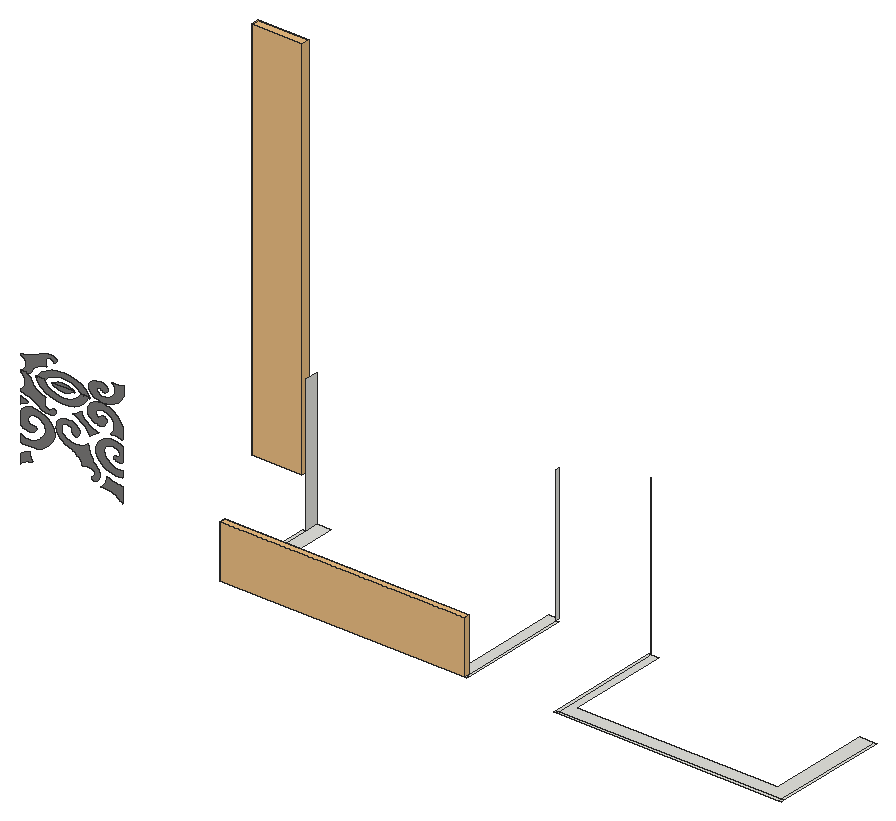
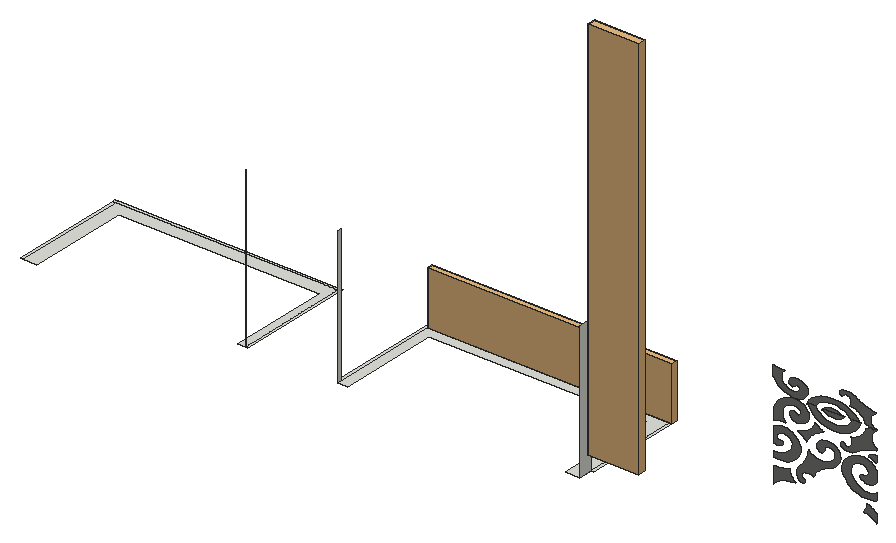
# SketchUp Ruby script. Lengths in inches.
U = 1.inch
M = Sketchup.active_model
def pt(a) = Geom::Point3d.new(a.map { |v| v * U })
def face(e, loops, mat)
  f = e.add_face(loops[0].map { |a| pt(a) })
  loops[1..].each { |l| e.add_face(l.map { |a| pt(a) }).erase! }
  f.material = f.back_material = mat if mat
  f
end
# faces: each face lists its corners as indices into pts; further lists are holes
def faces(e, pts, list, mat = nil) = list.each { |f| face(e, (f[0].is_a?(Array) ? f : [f]).map { |l| l.map { |i| pts[i] } }, mat) }
# xy, xz, yz: faces in a plane at the given z, y or x. An outline is a flat list of corners, or four numbers for a rectangle; further outlines are holes
def ring(l) = l.size == 4 ? [[l[0], l[1]], [l[2], l[1]], [l[2], l[3]], [l[0], l[3]]] : l.each_slice(2).to_a
def flat(e, list, mat, &to3) = list.each { |f| face(e, (f[0].is_a?(Array) ? f : [f]).map { |l| ring(l).map { |u, v| to3.(u, v) } }, mat) }
def xy(e, z, list, mat = nil) = flat(e, list, mat) { |x, y| [x, y, z] }
def xz(e, y, list, mat = nil) = flat(e, list, mat) { |x, z| [x, y, z] }
def yz(e, x, list, mat = nil) = flat(e, list, mat) { |y, z| [x, y, z] }
def lines(e, pts, list) = list.each { |a, b| e.add_line(pt(pts[a]), pt(pts[b])) }
# prism: a flat outline (further loops are holes) pulled along v
def prism(e, loops, v, mat = nil)
  f = face(e, loops, mat); d = Geom::Vector3d.new(v.map { |x| x * U })
  f.pushpull(f.normal.samedirection?(d) ? d.length : -d.length)
end
def box(e, o, s, mat = nil) = prism(e, [[o, [o[0] + s[0], o[1], o[2]], [o[0] + s[0], o[1] + s[1], o[2]], [o[0], o[1] + s[1], o[2]]]], [0, 0, s[2]], mat)
def at(x, y, z, deg = 0) = Geom::Transformation.translation(pt([x, y, z])) * Geom::Transformation.rotation(ORIGIN, Z_AXIS, deg.degrees)
def axes(o, x, y, z) = Geom::Transformation.new([*x, 0, *y, 0, *z, 0, *pt(o).to_a, 1])
def part(name) = M.definitions.add(name)
# library, detail: a bought-in or finely detailed component or shape, given as its bounding box
def library(name, o, s) = part(name).tap { |d| box(d.entities, o, s) }
def detail(e, o, s) = box(e.add_group.entities, o, s)
def put(e, d, t, mat = nil) = e.add_instance(d, t).tap { |i| i.material = mat if mat }
def group(e, t, mat = nil) = e.add_group.tap { |g| g.transformation = t; g.material = mat if mat }.entities
root = M.entities
M.materials.add("[0043_SaddleBrown]4").color = [124, 123, 122]
M.materials.add("[Granite Light Gray]").color = [149, 148, 144]
c1 = library("Scandinavian Door w/ Glass Wall\#2",[-41.94,78.85,0],[6.47,62.99,82.68])
c2 = library("Glass Railing",[0,0,0],[139.5,4.76,42])
xy(root,413.5,[[550.01,557.9375,742.44,559.875],[742.44,557.9375,744.38,559.875],[812.96,557.9375,814.89,559.875],[814.89,557.9375,990.19,559.875],[990.19,557.9375,992.12,559.875],
  [549.82,559.875,551.76,640.11],[551.76,559.875,742.44,559.875,742.44,651.03,734.59,651.03,734.59,570.83,563.08,570.83,563.08,651.03,551.76,651.03],[742.44,559.875,744.38,647.91],[812.96,559.875,814.89,651.03],[814.89,559.875,990.19,559.875,990.19,651.03,978.86,651.03,978.86,570.83,820.97,570.83,820.97,651.03,814.89,651.03],
  [990.19,559.875,992.12,651.03]])
xz(root,589.17,[[448.37,418.4,448.37,430.94,447.33,430.96,446.29,431.01,445.26,431.09,444.23,431.2,443.21,431.34,442.2,431.51,441.19,431.7,440.2,431.93,439.22,432.18,438.26,432.46,437.3125,432.77,436.38,433.11,436.28,432.33,436.12,431.56,435.91,430.79,435.64,430.03,435.32,429.29,434.95,428.55,434.53,427.83,434.05,427.13,433.53,426.44,432.96,425.78,432.34,425.14,431.68,424.52,433.34,424.625,435,424.61,436.65,424.48,438.27,424.22,439.85,423.85,441.36,423.36,442.8,422.76,444.15,422.0625,445.39,421.27,446.52,420.39,447.51,419.43],[367.98,418.5,368.5,419.14,369.09,419.74,369.74,420.3125,370.46,420.84,371.24,421.32,372.07,421.76,372.94,422.14,373.86,422.48,374.81,422.75,375.78,422.98,376.78,423.14,377.8,423.24,377.38,423.73,377,424.24,376.65,424.76,376.35,425.29,376.08,425.83,375.85,426.38,375.66,426.94,375.51,427.51,375.4,428.08,375.33,428.65,375.3,429.23,375.32,429.8,374.62,429.54,373.94,429.27,373.26,428.97,372.61,428.66,371.97,428.33,371.34,427.99,370.73,427.63,370.14,427.26,369.57,426.87,369.02,426.47,368.49,426.05,367.98,425.62],[426.05,427.2,426.61,427.23,427.15,427.32,427.68,427.46,428.16,427.66,428.61,427.9,429,428.18,429.33,428.51,429.6,428.86,429.79,429.24,429.91,429.63,429.94,430.04,430.16,430.71,430.3,431.38,430.38,432.07,430.39,432.76,430.32,433.44,430.19,434.125,429.99,434.8,429.73,435.46,429.39,436.1,428.99,436.72,428.54,437.33,428.02,437.9,427.08,438.91,426.21,439.95,425.41,441.02,424.67,442.11,424,443.22,423.41,444.36,422.88,445.51,422.43,446.68,422.05,447.86,421.75,449.05,421.52,450.26,421.37,451.46,420.4,450.57,419.28,449.77,418.03,449.08,416.66,448.52,415.2,448.09,413.68,447.8,412.12,447.66,410.54,447.66,408.98,447.8125,407.46,448.11,406.01,448.54,404.64,449.11,403.67,449.65,402.8,450.27,402.05,450.97,401.43,451.74,400.95,452.55,400.625,453.4,400.45,454.28,400.43,455.16,400.57,456.04,400.87,456.9,401.32,457.72,401.91,458.5,402.45,458.79,403.06,459.03,403.7,459.19,404.37,459.29,405.05,459.31,405.73,459.26,406.39,459.13,407.02,458.94,407.6,458.68,408.12,458.36,408.57,457.99,408.9375,457.57,408.82,457.28,408.73,456.98,408.68,456.67,408.66,456.37,408.67,456.06,408.72,455.75,408.8,455.45,408.91,455.16,409.06,454.87,409.24,454.59,409.45,454.32,409.68,454.0625,409.91,453.87,410.1875,453.7,410.49,453.5625,410.82,453.47,411.17,453.41,411.53,453.38,411.89,453.41,412.23,453.47,412.57,453.5625,412.87,453.7,413.14,453.87,413.375,454.0625,414.05,454.87,414.52,455.75,414.78,456.67,414.8125,457.61,414.625,458.54,414.22,459.4375,413.6,460.27,412.8,461.01,411.84,461.64,410.74,462.15,409.53,462.51,408.26,462.72,406.84,462.91,405.4,462.94,403.96,462.8125,402.58,462.53,401.26,462.1,400.05,461.53,398.98,460.83,398.07,460.03,397.33,459.13,396.79,458.17,396.47,457.15,396.36,456.12,396.24,454.92,396.31,453.72,396.54,452.53,396.94,451.37,397.51,450.24,398.24,449.16,399.12,448.14,400.14,447.19,401.29,446.32,402.56,445.55,403.93,444.87,405.4,444.3,406.79,443.78,408.12,443.1875,409.39,442.53,410.6,441.81,411.73,441.03,412.78,440.19,413.74,439.31,414.62,438.37,415.4,437.39,416.09,436.38,416.67,435.33,417.15,434.26,417.83,434.625,418.57,434.93,419.36,435.15,420.18,435.3,421.03,435.36,421.88,435.34,422.72,435.24,423.53,435.05,424.3,434.79,425.01,434.46,425.65,434.06,426.22,433.6,426.42,433.23,426.57,432.84,426.65,432.45,426.68,432.05,426.64,431.65,426.53,431.26,426.37,430.875,426.15,430.51,425.875,430.16,425.54,429.84,425.17,429.55,424.75,429.29,424.52,429.13,424.33,428.95,424.2,428.75,424.13,428.53,424.12,428.3,424.17,428.08,424.28,427.87,424.44,427.67,424.65,427.51,424.91,427.375,425.19,427.28,425.5,427.23],[374.59,433.3,376.85,433.36,379.09,433.62,381.26,434.07,383.35,434.7,385.3125,435.5,387.13,436.47,388.77,437.59,390.22,438.85,391.45,440.22,393.12,442.26,394.27,444.47,394.89,446.8,394.93,449.17,394.41,451.51,393.34,453.75,391.75,455.82,389.6875,457.67,387.21,459.23,384.41,460.46,381.35,461.32,378.13,461.79,376.97,461.63,375.83,461.4,374.74,461.08,373.6875,460.69,372.69,460.24,371.76,459.71,370.91,459.125,370.13,458.48,369.45,457.79,368.86,457.06,368.36,456.28,367.98,455.48,367.98,447.4,368.51,446.49,369.28,445.68,370.27,445,371.43,444.48,372.71,444.15,374.05,444,375.42,444.0625,376.73,444.32,377.95,444.76,379.01,445.37,379.88,446.13,380.52,447,380.62,447.21,380.67,447.42,380.67,447.64,380.63,447.86,380.55,448.07,380.42,448.27,380.26,448.46,380.06,448.62,379.82,448.76,379.57,448.88,379.29,448.97,378.99,449.02,378.26,448.93,377.53,448.94,376.81,449.05,376.125,449.25,375.5,449.54,374.97,449.9,374.53,450.33,374.22,450.81,374.03,451.32,373.97,451.85,374.06,452.38,374.27,452.89,374.45,453.55,374.78,454.18,375.24,454.77,375.82,455.29,376.51,455.75,377.28,456.12,378.13,456.4,379.03,456.57,379.96,456.65,380.89,456.62,381.81,456.48,382.68,456.24,384.03,455.45,385.22,454.53,386.22,453.51,387,452.39,387.5625,451.2,387.88,449.96,387.95,448.71,387.78,447.46,387.36,446.24,386.71,445.08,385.84,443.99,384.76,443.01,384.32,442.35,383.81,441.73,383.22,441.14,382.58,440.59,381.87,440.07,381.1,439.6,380.28,439.18,379.42,438.8125,378.51,438.49,377.57,438.23,376.61,438.03,375.625,437.88,374.92,437.82,374.22,437.8,373.51,437.83,372.8125,437.89,372.12,438,371.45,438.16,370.79,438.35,370.16,438.58,369.5625,438.85,368.99,439.15,368.46,439.48,367.98,439.85,367.98,434.28,370.12,433.76,372.34,433.44],[445.77,436.71,448.37,436.96,448.37,441.66,446.14,441.61,443.93,441.84,441.81,442.34,439.84,443.09,438.08,444.09,436.59,445.28,435.41,446.65,434.58,448.14,434.12,449.72,434.05,451.32,434.37,452.92,435.0625,454.45,435.86,455.1,436.81,455.63,437.88,456.03,439.04,456.27,440.24,456.35,441.45,456.27,442.6,456.02,443.68,455.625,444.625,455.09,445.42,454.43,446.03,453.68,446.43,452.86,446.5,452.53,446.49,452.1875,446.41,451.86,446.24,451.54,446,451.25,445.7,450.99,445.34,450.77,444.9375,450.61,444.5,450.49,444.04,450.43,443.57,450.42,443.11,450.48,442.87,450.4,442.64,450.31,442.43,450.19,442.23,450.06,442.06,449.92,441.9,449.77,441.78,449.6,441.67,449.42,441.6,449.24,441.55,449.06,441.53,448.87,441.54,448.68,441.9,448.29,442.34,447.9375,442.84,447.63,443.39,447.38,443.98,447.18,444.6,447.04,445.24,446.96,445.89,446.9375,446.54,446.98,447.18,447.09,447.79,447.25,448.37,447.47,448.37,459.11,447.3,459.72,446.15,460.23,444.91,460.64,443.62,460.9375,442.28,461.12,440.93,461.18,439.57,461.12,438.23,460.9375,436.9375,460.64,435.7,460.23,434.55,459.72,433.49,459.11,432.59,458.48,431.76,457.82,430.99,457.11,430.28,456.375,429.65,455.6,429.09,454.8,428.61,453.97,428.2,453.125,427.875,452.26,427.63,451.38,427.47,450.49,427.39,449.6,427.5,447.71,428.01,445.86,428.9,444.08,430.15,442.42,431.73,440.92,433.61,439.6,435.74,438.5,438.08,437.65,440.57,437.06,443.15,436.74],
  [422.47,457.23,423.02,457.6875,423.58,458.14,424.16,458.59,424.74,459.03,425.33,459.46,425.93,459.89,426.54,460.31,427.16,460.72,427.79,461.12,428.43,461.52,429.07,461.91,429.73,462.29,428.07,462.61,426.46,463.04,424.92,463.58,423.45,464.23,422.09,464.99,420.83,465.83,419.7,466.76,418.69,467.77,417.83,468.84,417.12,469.96,416.56,471.14,416.17,472.34,415.69,471.93,415.1875,471.54,414.66,471.16,414.12,470.79,413.5625,470.43,412.98,470.09,412.39,469.77,411.78,469.47,411.15,469.18,410.51,468.9,409.85,468.65,409.1875,468.41,410.75,467.83,412.25,467.18,413.6875,466.45,415.05,465.65,416.32,464.79,417.51,463.86,418.6,462.87,419.6,461.83,420.48,460.74,421.26,459.6,421.93,458.43],[367.98,460.92,368.39,461.25,368.83,461.57,369.28,461.88,369.76,462.17,370.25,462.45,370.76,462.71,371.28,462.95,371.82,463.18,372.37,463.39,372.93,463.58,373.51,463.75,374.09,463.91,373.71,464.24,373.3,464.55,372.86,464.84,372.39,465.11,371.9,465.35,371.38,465.56,370.85,465.76,370.3,465.92,369.73,466.05,369.15,466.16,368.57,466.24,367.98,466.28],[390.03,461.65,390.95,461.6875,391.86,461.8,392.75,461.98,393.6,462.23,393.91,462.34,394.2,462.47,394.47,462.62,394.73,462.79,394.96,462.96,395.18,463.16,395.37,463.36,395.54,463.58,395.68,463.8,395.79,464.03,395.88,464.27,395.94,464.52,395.97,464.75,395.95,464.99,395.9,465.23,395.82,465.46,395.69,465.6875,395.54,465.9,395.34,466.1,395.125,466.28,394.875,466.4375,394.6,466.58,394.3125,466.69,394,466.78,393.8125,466.54,393.61,466.29,393.39,466.06,392.93,465.6,392.68,465.38,392.42,465.17,392.15,464.96,391.87,464.77,391.58,464.57,391.28,464.39,390.97,464.21,390.55,464.28,390.14,464.375,389.74,464.5,389.36,464.65,389,464.83,388.67,465.03,388.36,465.26,388.09,465.5,387.86,465.77,387.66,466.04,387.49,466.33,387.37,466.63,387.23,467.11,387.12,467.58,387.04,468.0625,387,468.55,386.99,469.03,387.01,469.51,387.0625,469.99,387.15,470.47,387.27,470.95,387.42,471.42,387.6,471.88,387.82,472.34,386.35,472.75,384.9375,473.24,383.59,473.83,382.32,474.5,381.14,475.24,380.06,476.0625,379.08,476.95,378.21,477.9,377.47,478.89,376.85,479.94,376.36,481.01,376.01,482.12,375.63,482.3,375.26,482.48,374.89,482.68,374.54,482.88,374.1875,483.09,373.85,483.31,373.52,483.53,373.2,483.77,372.89,484.01,372.59,484.25,372.3,484.5,372.02,484.8,367.98,484.8,367.98,483.92,369.0625,483.03,369.98,482.05,370.71,480.99,371.24,479.87,371.5625,478.71,371.67,477.53,371.5625,476.35,371.24,475.1875,370.71,474.07,369.98,473.01,369.0625,472.02,367.98,471.14,367.98,469.95,369.45,469.73,370.9,469.45,372.33,469.11,373.74,468.72,375.11,468.27,376.44,467.77,377.73,467.21,378.98,466.61,380.1875,465.96,381.34,465.26,382.43,464.51,383.47,463.73,384.12,463.26,384.84,462.84,385.61,462.48,386.4375,462.18,387.3,461.94,388.19,461.77,389.11,461.68],[448.37,463.51,448.37,472.52,447.95,473.85,447.36,475.15,446.6,476.4,445.67,477.6,444.59,478.72,443.36,479.76,442,480.71,440.52,481.57,438.94,482.3125,437.26,482.95,435.5,483.46,433.68,483.85,432.01,483.91,430.35,483.79,428.74,483.49,427.2,483.03,425.77,482.4,424.49,481.63,423.38,480.73,422.47,479.72,421.78,478.625,421.32,477.47,421.1,476.28,421.13,475.07,421.08,474.3125,421.16,473.55,421.37,472.81,421.7,472.09,422.15,471.4,422.72,470.76,423.39,470.17,424.15,469.64,425,469.1875,425.91,468.81,426.89,468.51,427.9,468.31,428.58,468.02,429.31,467.82,430.09,467.71,430.875,467.7,431.65,467.78,432.4,467.96,433.09,468.22,433.71,468.57,434.24,468.99,434.67,469.47,434.97,469.99,435.15,470.54,435.55,470.95,435.84,471.4,436.03,471.88,436.09,472.38,436.04,472.88,435.87,473.36,435.58,473.81,435.2,474.23,434.72,474.59,434.16,474.88,433.53,475.1,432.87,475.24,432.64,474.99,432.39,474.75,432.14,474.52,431.875,474.29,431.6,474.07,431.3125,473.85,431.02,473.64,430.71,473.44,430.4,473.25,430.07,473.0625,429.74,472.88,429.4,472.71,429.03,472.88,428.69,473.08,428.37,473.31,428.09,473.55,427.85,473.82,427.66,474.1,427.5,474.4,427.39,474.71,427.33,475.02,427.32,475.34,427.35,475.66,427.43,475.97,427.72,476.6,428.14,477.18,428.6875,477.71,429.35,478.17,430.1,478.54,430.93,478.83,431.81,479.01,432.72,479.09,433.63,479.06,434.53,478.93,435.39,478.7,436.18,478.36,437.6,477.55,438.85,476.6,439.91,475.54,440.76,474.39,441.39,473.16,441.78,471.88,441.93,470.58,441.84,469.28,441.5,467.99,440.93,466.75,440.12,465.58,439.11,464.5,439.89,464.63,440.68,464.73,441.48,464.78,442.28,464.8,443.08,464.77,443.88,464.71,444.67,464.6,445.45,464.46,446.21,464.28,446.95,464.06,447.67,463.8],[401.21,472.34,406.03,472.75,410.59,473.95,414.65,475.88,417.98,478.43,420.41,481.46,421.8125,484.8,415.66,484.8,414.48,482.62,412.67,480.66,410.32,479.03,407.53,477.8,404.45,477.04,401.2,476.77,397.96,477.02,394.86,477.76,392.0625,478.97,389.69,480.59,387.86,482.53,386.65,484.8,380.49,484.8,381.93,481.37,384.38,478.35,387.74,475.82,391.8125,473.91,396.38,472.73],
  [401.52,480.9,403.29,481.02,404.99,481.375,406.5625,481.95,407.96,482.74,409.125,483.7,410.02,484.8,393.03,484.8,393.92,483.7,395.09,482.74,396.48,481.95,398.0625,481.375,399.76,481.02],[368.68,483.9,368.68,484.65,369.77,485.41,370.6875,486.24,371.42,487.15,371.95,488.1,372.27,489.09,372.375,490.1,372.27,491.1,371.95,492.09,371.42,493.05,370.6875,493.95,369.77,494.79,368.68,495.54,368.68,496.56,370.16,496.75,371.61,496.98,373.04,497.27,374.44,497.61,375.8125,497.99,377.15,498.41,378.44,498.89,379.69,499.4,380.89,499.96,382.04,500.55,383.14,501.1875,384.18,501.86,384.83,502.26,385.55,502.61,386.32,502.92,387.14,503.18,388.01,503.375,388.9,503.52,389.8125,503.6,390.73,503.63,391.66,503.59,392.56,503.5,393.45,503.34,394.31,503.13,394.61,503.04,394.9,502.92,395.18,502.8,395.43,502.66,395.67,502.51,395.88,502.34,396.08,502.17,396.24,501.98,396.39,501.79,396.5,501.59,396.59,501.39,396.65,501.18,396.67,500.98,396.66,500.78,396.61,500.57,396.52,500.375,396.4,500.1875,396.24,500.01,396.05,499.84,395.83,499.68,395.58,499.55,395.3125,499.43,395.02,499.33,394.71,499.25,394.52,499.46,394.31,499.67,394.1,499.87,393.87,500.07,393.63,500.26,393.38,500.44,393.125,500.625,392.85,500.8,392.58,500.97,392.29,501.13,391.99,501.29,391.68,501.44,391.26,501.38,390.84,501.3,390.44,501.2,390.06,501.07,389.71,500.91,389.375,500.74,389.07,500.55,388.8,500.34,388.5625,500.12,388.36,499.88,388.2,499.64,388.08,499.38,387.94,498.98,387.83,498.57,387.75,498.16,387.7,497.75,387.69,497.34,387.71,496.93,387.77,496.52,387.86,496.11,387.97,495.7,388.125,495.3,388.31,494.91,388.52,494.52,387.06,494.17,385.64,493.75,384.3,493.25,383.03,492.68,381.85,492.05,380.76,491.35,379.78,490.59,378.92,489.78,378.18,488.93,377.56,488.05,377.07,487.13,376.72,486.1875,376.34,486.04,375.96,485.88,375.24,485.54,374.89,485.36,374.23,484.98,373.91,484.78,373.6,484.58,373.3,484.37,373.01,484.16,372.73,483.9],[381.2,483.9,382.63,486.82,385.09,489.4,388.45,491.55,392.52,493.18,397.09,494.1875,401.92,494.52,406.74,494.17,411.3,493.14,415.35,491.5,418.6875,489.33,421.12,486.75,422.52,483.9,416.36,483.9,415.18,485.76,413.375,487.43,411.02,488.82,408.24,489.86,405.15,490.51,401.91,490.74,398.67,490.53,395.57,489.9,392.77,488.87,390.4,487.49,388.57,485.83,387.36,483.9],[393.73,483.9,394.63,484.84,395.8,485.66,397.19,486.33,398.77,486.82,400.47,487.125,402.23,487.23,403.99,487.125,405.69,486.82,407.27,486.33,408.67,485.66,409.83,484.84,410.73,483.9],[432.72,484.66,431.0625,484.76,429.44,485.02,427.9,485.41,426.48,485.95,425.2,486.6,424.09,487.37,423.18,488.23,422.48,489.16,422.02,490.15,421.8,491.16,421.83,492.1875,421.79,492.84,421.87,493.48,422.08,494.12,422.41,494.73,422.86,495.32,423.43,495.87,424.09,496.37,424.86,496.82,425.7,497.21,426.62,497.53,427.59,497.78,428.61,497.95,429.29,498.2,430.02,498.37,430.79,498.46,431.58,498.48,432.36,498.4,433.11,498.25,433.8,498.02,434.42,497.73,434.95,497.37,435.375,496.96,435.68,496.52,435.86,496.05,436.25,495.7,436.55,495.32,436.73,494.91,436.8,494.48,436.75,494.0625,436.58,493.65,436.29,493.26,435.9,492.91,435.42,492.6,434.86,492.35,434.24,492.17,433.58,492.05,433.34,492.26,433.1,492.46,432.85,492.66,432.58,492.86,432.3,493.05,432.02,493.23,431.72,493.41,431.42,493.58,430.78,493.9,430.45,494.05,430.11,494.2,429.74,494.05,429.39,493.89,429.08,493.7,428.8,493.49,428.5625,493.26,428.36,493.02,428.21,492.76,428.1,492.5,428.04,492.23,428.02,491.96,428.06,491.69,428.14,491.43,428.42,490.89,428.85,490.39,429.4,489.94,430.06,489.55,430.81,489.23,431.64,488.99,432.52,488.83,433.43,488.77,434.34,488.79,435.24,488.9,436.09,489.1,436.89,489.39,438.3,490.08,439.55,490.89,440.61,491.79,441.47,492.77,442.1,493.82,442.49,494.91,442.64,496.02,442.55,497.13,442.21,498.22,441.63,499.28,440.83,500.28,439.81,501.2,440.6,501.09,441.39,501.01,442.1875,500.96,442.99,500.95,443.79,500.97,444.59,501.02,445.38,501.11,446.16,501.23,446.92,501.39,447.66,501.57,448.38,501.79,449.07,502.04,449.07,494.37,448.66,493.23,448.07,492.125,447.3,491.06,446.38,490.04,445.3,489.08,444.07,488.2,442.71,487.38,441.23,486.66,439.64,486.02,437.96,485.48,436.21,485.04,434.39,484.71]],"[0043_SaddleBrown]4")
xz(root,651.03,[[814.68,413.5,814.89,538.1875]])
yz(root,551.76,[[640.11,413.5,651.03,520.4375]])
yz(root,742.44,[[647.91,413.5,651.03,520.4375]])
p = [[367.98,589.17,469.95],[367.98,589.17,466.28]]
lines(root,p,[[0,1]])
put(root,c1,axes([446.25,621.1,440.32],[0,-1,0],[0.63229,0,0],[0,0,3.672]))
put(root,c2,axes([550.01,557.9375,413.5],[1.37946,0,0],[0,1,0],[0,0,1]),"[Granite Light Gray]")
